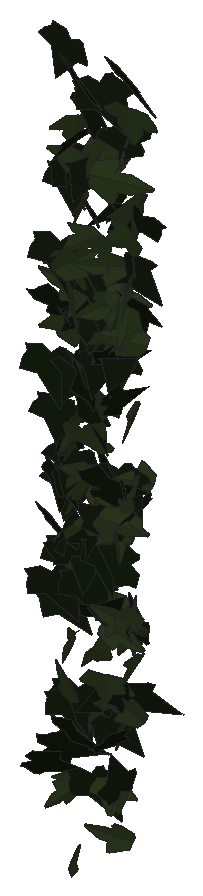
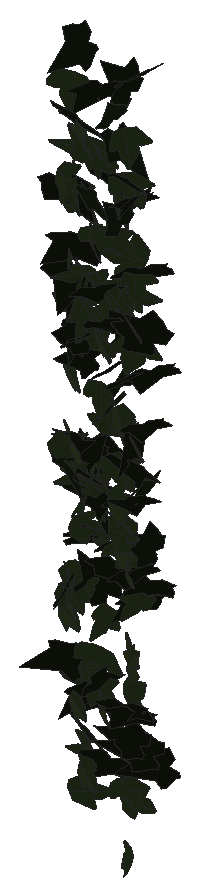
# SketchUp Ruby script. Lengths in inches.
U = 1.inch
M = Sketchup.active_model
def pt(a) = Geom::Point3d.new(a.map { |v| v * U })
def face(e, loops, mat)
  f = e.add_face(loops[0].map { |a| pt(a) })
  loops[1..].each { |l| e.add_face(l.map { |a| pt(a) }).erase! }
  f.material = f.back_material = mat if mat
  f
end
# faces: each face lists its corners as indices into pts; further lists are holes
def faces(e, pts, list, mat = nil) = list.each { |f| face(e, (f[0].is_a?(Array) ? f : [f]).map { |l| l.map { |i| pts[i] } }, mat) }
# xy, xz, yz: faces in a plane at the given z, y or x. An outline is a flat list of corners, or four numbers for a rectangle; further outlines are holes
def ring(l) = l.size == 4 ? [[l[0], l[1]], [l[2], l[1]], [l[2], l[3]], [l[0], l[3]]] : l.each_slice(2).to_a
def flat(e, list, mat, &to3) = list.each { |f| face(e, (f[0].is_a?(Array) ? f : [f]).map { |l| ring(l).map { |u, v| to3.(u, v) } }, mat) }
def xy(e, z, list, mat = nil) = flat(e, list, mat) { |x, y| [x, y, z] }
def xz(e, y, list, mat = nil) = flat(e, list, mat) { |x, z| [x, y, z] }
def yz(e, x, list, mat = nil) = flat(e, list, mat) { |y, z| [x, y, z] }
def lines(e, pts, list) = list.each { |a, b| e.add_line(pt(pts[a]), pt(pts[b])) }
# prism: a flat outline (further loops are holes) pulled along v
def prism(e, loops, v, mat = nil)
  f = face(e, loops, mat); d = Geom::Vector3d.new(v.map { |x| x * U })
  f.pushpull(f.normal.samedirection?(d) ? d.length : -d.length)
end
def box(e, o, s, mat = nil) = prism(e, [[o, [o[0] + s[0], o[1], o[2]], [o[0] + s[0], o[1] + s[1], o[2]], [o[0], o[1] + s[1], o[2]]]], [0, 0, s[2]], mat)
def at(x, y, z, deg = 0) = Geom::Transformation.translation(pt([x, y, z])) * Geom::Transformation.rotation(ORIGIN, Z_AXIS, deg.degrees)
def axes(o, x, y, z) = Geom::Transformation.new([*x, 0, *y, 0, *z, 0, *pt(o).to_a, 1])
def part(name) = M.definitions.add(name)
# library, detail: a bought-in or finely detailed component or shape, given as its bounding box
def library(name, o, s) = part(name).tap { |d| box(d.entities, o, s) }
def detail(e, o, s) = box(e.add_group.entities, o, s)
def put(e, d, t, mat = nil) = e.add_instance(d, t).tap { |i| i.material = mat if mat }
def group(e, t, mat = nil) = e.add_group.tap { |g| g.transformation = t; g.material = mat if mat }.entities
root = M.entities
M.materials.add("1026 AP 7946 SUNNY SIDE UP").color = [254, 231, 186]
M.materials.add("efeu1").color = [18, 25, 13]
M.materials.add("efeu2").color = [43, 57, 29]
c1 = part("ivyleaf_10")
p = [[0,0.5,-0.03],[-0.0625,2.02,-0.43],[-0.19,2.01,-0.46],[-0.54,1.05,-0.29],[-0.52,0.625,-0.18],[-0.83,0.76,-0.28],
  [-1.16,0.64,-0.33],[-1.15,0.33,-0.24],[-0.77,-0.39,0.02],[-0.3,-0.51,0.16],[0.04,-0.48,0.23],[-0.02,2.01,-0.4375],
  [-0.06,2.01,-0.43],[0.04,-0.49,0.23],[0.67,-0.49,0.14],[1.38,0.36,-0.2],[1.375,0.51,-0.24],[0.81,0.65,-0.19],
  [0.62,0.59,-0.15],[0.6,1.09,-0.28],[0.5,1.23,-0.31]]
faces(c1.entities,p,[[0,1,2,3,4,5,6,7,8,9,10],[11,12,0,13,14,15,16,17,18,19,20]],"efeu2")
c2 = part("ivyleaf_9")
p = [[1.54,2.16,1.25],[1.36,2.04,1.19],[-0.21,0.99,0.68],[-0.71,1.11,0.82],[-0.85,0.86,0.67],[-0.8,0.17,0.21],
  [-0.9,-0.01,0.1],[-0.67,-0.16,-0.02],[-0.08,-0.08,-0.05],[-0.03,-0.6,-0.4],[0.65,-0.88,-0.66],[0.83,-0.6,-0.49],
  [1.29,-0.42,-0.43],[1.8125,-0.07,-0.26],[1.21,0.44,0.15]]
faces(c2.entities,p,[[0,1,2,3,4,5,6,7,8,9,10,11,12,13,14]],"efeu1")
put(root,c1,axes([112.04,211.58,259.63],[-0.02218,-0.00666,0.26985],[0.14975,-0.24455,-0.00255],[0.38389,0.09501,0.01659]),"1026 AP 7946 SUNNY SIDE UP")
put(root,c2,axes([113.1,211.2,254.04],[0.15391,0.18308,0.14544],[0.11528,0.11962,-0.21306],[-0.34372,0.1221,-0.00633]),"1026 AP 7946 SUNNY SIDE UP")
put(root,c2,axes([113.43,211.23,253.19],[-0.30936,0.08367,-0.17603],[-0.22814,0.09407,0.2195],[0.19456,0.24335,-0.02252]),"1026 AP 7946 SUNNY SIDE UP")
put(root,c2,axes([112.72,211.41,259],[0.10094,0.00315,0.26449],[0.3707,-0.10549,-0.06002],[0.15983,0.24268,-0.02783]),"1026 AP 7946 SUNNY SIDE UP")
put(root,c2,axes([111.45,211.28,253.05],[0.27439,0.08812,0.17342],[0.25302,0.05173,-0.20003],[-0.15756,0.23652,-0.01922]),"1026 AP 7946 SUNNY SIDE UP")
put(root,c2,axes([111.625,211.52,261.22],[-0.10121,-0.2792,-0.08746],[0.02947,0.08118,-0.2947],[0.4572,-0.06704,-0.00036]),"1026 AP 7946 SUNNY SIDE UP")
put(root,c1,axes([113.27,211.5,252.01],[-0.09095,-0.01215,-0.2455],[-0.36534,-0.05265,0.06058],[-0.08495,0.23943,0.00233]),"1026 AP 7946 SUNNY SIDE UP")
put(root,c1,axes([113.06,211.34,258.47],[-0.13431,-0.07695,-0.25617],[0.36398,0.09625,-0.11223],[0.18576,-0.24423,0.03468]),"1026 AP 7946 SUNNY SIDE UP")
put(root,c1,axes([112.02,211.51,262.68],[-0.19608,0.22953,-0.16457],[0.09734,-0.14937,-0.26957],[-0.43001,-0.13848,0.01402]),"1026 AP 7946 SUNNY SIDE UP")
put(root,c2,axes([112.35,211.26,257.6],[-0.41504,0.13352,-0.08424],[-0.09726,0.05992,0.30403],[0.22684,0.26998,-0.02377]),"1026 AP 7946 SUNNY SIDE UP")
put(root,c2,axes([111.7,211.46,256.84],[-0.11315,-0.17882,-0.1991],[0.18009,0.15799,-0.19464],[0.3715,-0.13105,0.03372]),"1026 AP 7946 SUNNY SIDE UP")
put(root,c2,axes([111.68,211.64,258.74],[0.02999,-0.21354,0.17123],[0.00604,-0.16761,-0.22166],[0.42663,0.01739,-0.0089]),"1026 AP 7946 SUNNY SIDE UP")
put(root,c1,axes([113.03,211.4375,256.21],[0.11464,0.0422,0.24505],[0.36719,0.05035,-0.08273],[-0.09583,0.2434,-0.02384]),"1026 AP 7946 SUNNY SIDE UP")
put(root,c1,axes([113.3,211.4,253.03],[0.19212,-0.17785,-0.15897],[-0.15254,0.11914,-0.22135],[0.33622,0.15568,-0.00959]),"1026 AP 7946 SUNNY SIDE UP")
put(root,c2,axes([112.6875,211.5625,257.63],[0.04379,-0.2629,-0.01141],[-0.00693,0.00917,-0.27228],[0.4136,0.02799,-0.00336]),"1026 AP 7946 SUNNY SIDE UP")
put(root,c1,axes([113.31,211.55,262.59],[0.39846,-0.1214,0.07714],[0.08661,-0.05904,-0.28833],[0.20751,0.25776,-0.02779]),"1026 AP 7946 SUNNY SIDE UP")
put(root,c1,axes([113.01,211.58,263.48],[0.02748,0.00647,-0.26841],[-0.36284,-0.12107,-0.01975],[-0.19061,0.23141,-0.0011]),"1026 AP 7946 SUNNY SIDE UP")
put(root,c1,axes([113.32,211.51,258.93],[0.22626,-0.23331,-0.07497],[0.0778,-0.05332,0.28172],[-0.3757,-0.15155,0.01319]),"1026 AP 7946 SUNNY SIDE UP")
put(root,c2,axes([113.15,211.27,260.85],[0.06119,0.07554,0.25029],[0.27377,0.17072,-0.08257],[-0.29084,0.1766,-0.02506]),"1026 AP 7946 SUNNY SIDE UP")
put(root,c1,axes([113.34,211.5625,256.36],[-0.17491,-0.06534,-0.24772],[-0.35927,-0.07733,0.13028],[-0.15494,0.25306,-0.02244]),"1026 AP 7946 SUNNY SIDE UP")
put(root,c2,axes([112.3,211.62,257.53],[-0.10673,-0.26645,0.00292],[0.0045,-0.00521,-0.28327],[0.419,-0.06782,0.00378]),"1026 AP 7946 SUNNY SIDE UP")
put(root,c2,axes([112.42,211.51,256.98],[-0.164,-0.16956,-0.1863],[0.16946,0.14451,-0.20386],[0.34981,-0.1495,0.01142]),"1026 AP 7946 SUNNY SIDE UP")
put(root,c1,axes([113.48,211.6,262.07],[0.05756,0.07026,0.26662],[-0.25577,-0.20135,0.07896],[0.33449,-0.16605,0.01449]),"1026 AP 7946 SUNNY SIDE UP")
put(root,c2,axes([112.01,211.66,266.95],[0.14269,-0.16151,0.25112],[0.15557,-0.22424,-0.1916],[0.43395,0.1335,-0.01389]),"1026 AP 7946 SUNNY SIDE UP")
put(root,c1,axes([112.77,211.36,255.77],[-0.09376,-0.18861,-0.18934],[0.09541,0.17241,-0.20272],[0.40174,-0.08496,0.00396]),"1026 AP 7946 SUNNY SIDE UP")
put(root,c1,axes([113.45,211.6,260.7],[0.18456,-0.24275,0.09962],[0.05247,-0.09274,-0.27814],[0.40832,0.12164,-0.00929]),"1026 AP 7946 SUNNY SIDE UP")
put(root,c1,axes([112.11,211.31,263.27],[-0.0451,-0.13676,0.28314],[0.07044,0.272,0.14544],[-0.47864,0.05291,-0.00528]),"1026 AP 7946 SUNNY SIDE UP")
put(root,c1,axes([113.51,211.61,255.68],[0.04975,-0.21554,0.11849],[0.01456,-0.11607,-0.225],[0.38479,0.03226,-0.0068]),"1026 AP 7946 SUNNY SIDE UP")
put(root,c1,axes([112.85,211.45,265.29],[-0.00563,-0.0652,-0.31993],[0.49465,0.0372,-0.01158],[0.06094,-0.30796,0.06443]),"1026 AP 7946 SUNNY SIDE UP")
put(root,c1,axes([112.84,211.69,262.6],[0.08409,0.05383,-0.28802],[-0.25768,-0.22719,-0.0786],[-0.36668,0.172,-0.01082]),"1026 AP 7946 SUNNY SIDE UP")
put(root,c1,axes([112.4,211.61,259.1],[-0.22738,-0.19886,0.1324],[-0.08747,-0.1192,-0.25297],[0.36288,-0.15334,0.02199]),"1026 AP 7946 SUNNY SIDE UP")
put(root,c1,axes([112.5,211.53,259.78],[-0.38482,-0.04109,0.09426],[0.13978,0.0242,0.25564],[-0.07376,0.26024,-0.00732]),"1026 AP 7946 SUNNY SIDE UP")
put(root,c1,axes([111.93,211.62,259.73],[0.22835,-0.19183,0.08979],[0.06406,-0.07963,-0.24787],[0.32577,0.15012,-0.01419]),"1026 AP 7946 SUNNY SIDE UP")
put(root,c1,axes([113.4,211.5,264.22],[-0.24453,0.03139,0.20914],[-0.32189,-0.00541,-0.16087],[-0.02323,-0.25553,0.02758]),"1026 AP 7946 SUNNY SIDE UP")
put(root,c1,axes([112.97,211.57,252.9375],[0.3752,0.04405,0.02018],[0.03601,-0.01795,-0.24907],[-0.06653,0.23872,-0.021]),"1026 AP 7946 SUNNY SIDE UP")
put(root,c2,axes([112.64,211.53,256.32],[0.33869,0.12977,0.02203],[-0.04503,0.00767,0.25817],[0.20165,-0.21625,0.02066]),"1026 AP 7946 SUNNY SIDE UP")
put(root,c1,axes([113.1,211.6,258.12],[-0.02846,0.22322,-0.12106],[0.01378,-0.11846,-0.23141],[-0.39735,-0.0201,0.00065]),"1026 AP 7946 SUNNY SIDE UP")
put(root,c1,axes([113.22,211.59,258.7],[0.41399,-0.0452,-0.10964],[-0.17161,-0.01167,-0.27377],[0.05891,0.28364,-0.02703]),"1026 AP 7946 SUNNY SIDE UP")
put(root,c2,axes([111.79,211.52,256.48],[0.04527,-0.19567,-0.19128],[0.03036,0.18664,-0.19966],[0.42186,0.00757,0.03489]),"1026 AP 7946 SUNNY SIDE UP")
put(root,c2,axes([111.95,211.74,261.82],[-0.01217,-0.13586,0.2379],[0.13872,-0.22022,-0.13128],[0.39891,0.07244,0.05291]),"1026 AP 7946 SUNNY SIDE UP")
put(root,c2,axes([112.26,211.78,260.69],[-0.11172,-0.05878,0.27334],[-0.07183,-0.26809,-0.07526],[0.42175,-0.06123,0.05959]),"1026 AP 7946 SUNNY SIDE UP")
put(root,c2,axes([112.95,211.47,258.21],[-0.34215,0.02034,0.17623],[0.27063,0.01926,0.22344],[0.00633,0.27605,-0.02695]),"1026 AP 7946 SUNNY SIDE UP")
put(root,c1,axes([113.44,211.59,264.4],[-0.2305,0.2057,0.05092],[0.06399,-0.03016,0.25955],[0.326,0.15135,-0.01494]),"1026 AP 7946 SUNNY SIDE UP")
put(root,c2,axes([111.68,211.68,260.17],[-0.1405,-0.23919,-0.0491],[0.02635,0.04317,-0.2628],[0.38218,-0.09091,0.00007]),"1026 AP 7946 SUNNY SIDE UP")
put(root,c1,axes([113.1,211.62,262.25],[0.30775,-0.2433,-0.0362],[-0.05585,0.01468,-0.32103],[0.38217,0.19806,-0.01776]),"1026 AP 7946 SUNNY SIDE UP")
put(root,c2,axes([112.33,211.42,262.29],[-0.10707,0.2184,0.15919],[-0.08456,0.14372,-0.23472],[-0.41094,-0.08648,0.00682]),"1026 AP 7946 SUNNY SIDE UP")
put(root,c2,axes([113.08,211.62,259.32],[-0.15925,-0.1492,-0.20461],[0.23664,0.13265,-0.18172],[0.30941,-0.17824,0.03367]),"1026 AP 7946 SUNNY SIDE UP")
put(root,c2,axes([111.64,211.5,253.3],[0.18327,0.02019,0.24018],[0.36751,-0.00006,-0.12043],[-0.01412,0.26055,-0.01711]),"1026 AP 7946 SUNNY SIDE UP")
put(root,c1,axes([113.4,211.7,256.17],[-0.10942,-0.20613,0.11958],[-0.04406,-0.11418,-0.22461],[0.37027,-0.0745,0.00861]),"1026 AP 7946 SUNNY SIDE UP")
put(root,c1,axes([112.71,211.7,254.41],[-0.09429,-0.22143,0.11188],[-0.032,-0.10824,-0.23682],[0.38735,-0.06284,0.00767]),"1026 AP 7946 SUNNY SIDE UP")
put(root,c2,axes([113.07,211.57,267.5],[0.44822,-0.12414,-0.05396],[-0.08868,-0.00043,-0.31945],[0.19194,0.2897,-0.02159]),"1026 AP 7946 SUNNY SIDE UP")
put(root,c2,axes([112.08,211.78,260.98],[-0.16612,-0.20449,0.09169],[-0.04367,-0.08694,-0.23718],[0.34869,-0.10831,0.01398]),"1026 AP 7946 SUNNY SIDE UP")
put(root,c1,axes([112.25,211.65,264.52],[0.10419,-0.24391,0.01775],[-0.00015,-0.01931,-0.26044],[0.38464,0.06606,-0.00491]),"1026 AP 7946 SUNNY SIDE UP")
put(root,c1,axes([112.8,211.59,255.02],[-0.45319,-0.01634,-0.04731],[0.07441,-0.03017,-0.29569],[0.01777,-0.29027,0.03167]),"1026 AP 7946 SUNNY SIDE UP")
put(root,c2,axes([113.15,211.77,257.41],[-0.13407,-0.24512,-0.14438],[-0.08108,-0.12894,0.26655],[-0.43541,0.09949,-0.00518]),"1026 AP 7946 SUNNY SIDE UP")
put(root,c1,axes([111.98,211.56,257.32],[0.11102,-0.01553,-0.26424],[0.40225,0.0283,0.07097],[0.03653,-0.26444,0.02154]),"1026 AP 7946 SUNNY SIDE UP")
put(root,c2,axes([112.49,211.61,252.97],[-0.13245,-0.12284,-0.22839],[0.23434,0.16405,-0.1515],[0.32117,-0.17036,0.01635]),"1026 AP 7946 SUNNY SIDE UP")
put(root,c1,axes([111.86,211.76,252.4],[-0.05228,-0.11875,0.2008],[-0.05789,-0.19229,-0.12785],[0.35511,-0.04883,0.00872]),"1026 AP 7946 SUNNY SIDE UP")
put(root,c2,axes([112.36,211.73,260.3],[0.10743,-0.25465,0.03821],[0.00687,-0.03871,-0.27178],[0.40492,0.06822,-0.00553]),"1026 AP 7946 SUNNY SIDE UP")
put(root,c2,axes([111.82,211.625,258.79],[0.17564,-0.21305,-0.08843],[-0.0805,0.06858,-0.24707],[0.35136,0.12221,-0.0124]),"1026 AP 7946 SUNNY SIDE UP")
put(root,c1,axes([113.05,211.75,263.01],[0.32754,-0.14504,0.1643],[0.18119,-0.11386,-0.26105],[0.28762,0.23691,-0.02265]),"1026 AP 7946 SUNNY SIDE UP")
put(root,c1,axes([112.53,211.77,254.03],[0.14231,-0.07996,0.21829],[0.20913,-0.16653,-0.12397],[0.28906,0.15984,-0.01777]),"1026 AP 7946 SUNNY SIDE UP")
put(root,c1,axes([112.44,211.71,263.8125],[-0.22213,-0.08699,0.19607],[-0.22333,-0.12958,-0.16995],[0.24261,-0.19894,0.02308]),"1026 AP 7946 SUNNY SIDE UP")
put(root,c1,axes([113.34,211.62,266.66],[-0.46388,-0.00019,0.01272],[-0.01929,-0.0293,-0.30259],[0.00222,-0.29381,0.02843]),"1026 AP 7946 SUNNY SIDE UP")
put(root,c2,axes([112.04,211.73,259.29],[-0.36718,-0.09221,-0.12032],[0.18076,0.02469,-0.25787],[0.14757,-0.25969,0.01649]),"1026 AP 7946 SUNNY SIDE UP")
put(root,c1,axes([112.09,211.62,262.73],[-0.06583,-0.01384,-0.26069],[-0.39033,0.05347,0.03962],[0.0796,0.25077,-0.02129]),"1026 AP 7946 SUNNY SIDE UP")
put(root,c2,axes([112.69,211.84,254.58],[0.0069,-0.10624,-0.22872],[0.13024,-0.20783,0.10321],[-0.36353,-0.07648,0.03263]),"1026 AP 7946 SUNNY SIDE UP")
put(root,c2,axes([111.66,211.73,263.39],[-0.12418,-0.27694,-0.09736],[0.0577,0.0861,-0.29595],[0.45568,-0.08637,0.01094]),"1026 AP 7946 SUNNY SIDE UP")
put(root,c2,axes([112.24,211.83,266.34],[-0.00785,-0.21064,0.1636],[0.05608,-0.15911,-0.21557],[0.41214,0.01764,0.03245]),"1026 AP 7946 SUNNY SIDE UP")
put(root,c2,axes([112.24,211.65,265.9],[-0.15795,0.25238,-0.15154],[0.06135,-0.1441,-0.28026],[-0.45637,-0.10672,0.01477]),"1026 AP 7946 SUNNY SIDE UP")
put(root,c2,axes([113.5625,211.5,258.75],[-0.09048,0.25111,0.084],[-0.03984,0.07635,-0.26485],[-0.41254,-0.06245,0.00715]),"1026 AP 7946 SUNNY SIDE UP")
put(root,c1,axes([113.46,211.62,254.52],[-0.19768,0.01268,-0.22864],[-0.33636,0.06276,0.12885],[0.09551,0.24729,-0.01944]),"1026 AP 7946 SUNNY SIDE UP")
put(root,c1,axes([112.33,211.76,262.46],[-0.15523,-0.15216,0.15867],[-0.09617,-0.14376,-0.1865],[0.32758,-0.11431,0.02044]),"1026 AP 7946 SUNNY SIDE UP")
put(root,c2,axes([112.92,211.83,261.61],[-0.14352,-0.26704,0.04553],[-0.00759,-0.04662,-0.29081],[0.42594,-0.09081,0.01016]),"1026 AP 7946 SUNNY SIDE UP")
put(root,c2,axes([111.38,211.75,257.73],[0.23222,-0.15976,0.16517],[0.15513,-0.12806,-0.22456],[0.32143,0.17722,-0.01095]),"1026 AP 7946 SUNNY SIDE UP")
put(root,c2,axes([113.01,211.61,258.95],[0.13801,-0.14852,0.23433],[-0.11441,0.21837,0.17643],[-0.4127,-0.1102,0.02945]),"1026 AP 7946 SUNNY SIDE UP")
put(root,c1,axes([112.2,211.5625,257.93],[-0.16153,-0.12621,-0.18159],[0.20611,0.11821,-0.16588],[0.27036,-0.16552,0.01797]),"1026 AP 7946 SUNNY SIDE UP")
put(root,c1,axes([112.93,211.84,265.74],[-0.09131,0.01975,-0.27374],[0.11318,-0.26079,-0.03769],[-0.40357,-0.07761,0.05136]),"1026 AP 7946 SUNNY SIDE UP")
put(root,c2,axes([111.99,211.49,259.73],[0.0301,-0.04196,-0.29131],[-0.27789,0.22071,-0.04481],[0.35283,0.17741,-0.01044]),"1026 AP 7946 SUNNY SIDE UP")
put(root,c2,axes([112.9375,211.59,254.27],[0.022,-0.15416,-0.23039],[-0.02336,0.22228,-0.15814],[0.42533,0.02018,0.00323]),"1026 AP 7946 SUNNY SIDE UP")
put(root,c2,axes([111.74,211.73,253.57],[0.20267,-0.0685,0.20722],[0.24676,-0.12859,-0.14918],[0.22612,0.20172,-0.02293]),"1026 AP 7946 SUNNY SIDE UP")
put(root,c1,axes([113.49,211.84,259.16],[0.02272,0.09849,0.24176],[-0.06889,-0.23001,0.10113],[0.39338,-0.04597,0.00374]),"1026 AP 7946 SUNNY SIDE UP")
put(root,c1,axes([112,211.6,257.61],[0.20312,0.141,0.18435],[0.2213,0.11121,-0.19516],[-0.28044,0.18988,-0.02048]),"1026 AP 7946 SUNNY SIDE UP")
put(root,c1,axes([111.8,211.77,255.3],[0.06487,-0.20424,-0.10409],[0.0715,-0.09205,0.21272],[-0.35027,-0.05661,0.02414]),"1026 AP 7946 SUNNY SIDE UP")
put(root,c1,axes([112.02,211.6,254.48],[-0.23971,0.1351,-0.17683],[-0.18257,0.12829,0.21007],[0.29206,0.19108,-0.01383]),"1026 AP 7946 SUNNY SIDE UP")
put(root,c2,axes([112.88,211.7,261.5],[0.32634,0.20053,0.10751],[-0.14592,-0.05191,0.29584],[0.32322,-0.22591,0.02501]),"1026 AP 7946 SUNNY SIDE UP")
put(root,c1,axes([113.3,211.62,256.25],[0.23302,-0.18452,0.14097],[-0.11286,0.1188,0.24395],[-0.34417,-0.16389,0.01544]),"1026 AP 7946 SUNNY SIDE UP")
put(root,c1,axes([111.71,211.61,256.52],[0.11219,0.20213,0.14086],[0.09407,0.12239,-0.21969],[-0.37097,0.09216,-0.01311]),"1026 AP 7946 SUNNY SIDE UP")
put(root,c2,axes([112.8,211.66,258.41],[0.18371,-0.00878,-0.22961],[-0.34938,-0.02589,-0.11912],[-0.0297,0.25026,-0.01889]),"1026 AP 7946 SUNNY SIDE UP")
put(root,c1,axes([112.1,211.92,258.55],[0.07732,-0.15533,0.25408],[0.07427,-0.24347,-0.16849],[0.45344,0.06637,-0.01573]),"1026 AP 7946 SUNNY SIDE UP")
put(root,c1,axes([111.76,211.9,255.26],[0.0254,0.00619,0.27112],[0.20216,-0.23023,-0.00389],[0.36114,0.12844,-0.01689]),"1026 AP 7946 SUNNY SIDE UP")
put(root,c1,axes([112.08,211.56,251.05],[0.05657,-0.05491,0.23782],[-0.17548,0.20249,0.06863],[-0.32981,-0.11716,0.00428]),"1026 AP 7946 SUNNY SIDE UP")
put(root,c1,axes([112.01,211.74,266.02],[-0.18595,-0.2516,-0.00307],[0.01295,-0.00215,-0.28628],[0.39541,-0.11825,0.00793]),"1026 AP 7946 SUNNY SIDE UP")
put(root,c1,axes([112.17,211.73,260.23],[0.02099,-0.26389,-0.02971],[-0.0109,0.02702,-0.27199],[0.41702,0.01399,-0.00562]),"1026 AP 7946 SUNNY SIDE UP")
put(root,c2,axes([113.49,211.73,264.59],[0.11559,0.08063,-0.24591],[-0.28945,-0.15329,-0.11243],[-0.2715,0.19775,0.01516]),"1026 AP 7946 SUNNY SIDE UP")
put(root,c1,axes([113.2,211.88,256.06],[0.12437,-0.05986,0.2357],[0.24008,-0.17178,-0.10153],[0.28466,0.17103,-0.01735]),"1026 AP 7946 SUNNY SIDE UP")
put(root,c2,axes([111.6875,211.9375,267.43],[-0.13555,-0.23887,0.11899],[-0.01089,-0.12079,-0.26033],[0.418,-0.08061,0.03181]),"1026 AP 7946 SUNNY SIDE UP")
put(root,c2,axes([111.78,211.83,264.84],[-0.07589,-0.2476,-0.04357],[0.03533,0.03721,-0.25922],[0.39302,-0.05115,0.01489]),"1026 AP 7946 SUNNY SIDE UP")
put(root,c2,axes([113.4,211.54,261.47],[-0.11009,0.03489,-0.26612],[-0.3005,0.17533,0.07873],[0.27919,0.20247,-0.0202]),"1026 AP 7946 SUNNY SIDE UP")
put(root,c1,axes([111.78,211.74,263.25],[-0.16261,-0.22445,-0.03732],[0.04853,0.02416,-0.25379],[0.35386,-0.10645,0.01766]),"1026 AP 7946 SUNNY SIDE UP")
put(root,c1,axes([113.34,211.86,264.8],[0.01455,-0.24604,0.12115],[0.01216,-0.11878,-0.25433],[0.42958,0.0117,0.0031]),"1026 AP 7946 SUNNY SIDE UP")
put(root,c1,axes([112.875,211.7,262.03],[-0.24308,-0.19912,-0.09224],[0.11178,0.05637,-0.25852],[0.32382,-0.16893,0.02]),"1026 AP 7946 SUNNY SIDE UP")
put(root,c1,axes([112.54,211.81,261.73],[0.11753,-0.23624,0.04104],[0.0123,-0.04071,-0.25545],[0.37686,0.075,-0.00446]),"1026 AP 7946 SUNNY SIDE UP")
put(root,c1,axes([112.19,211.85,262.68],[-0.01921,-0.03916,0.24968],[0.35167,-0.10238,-0.00602],[0.16005,0.22026,0.0432]),"1026 AP 7946 SUNNY SIDE UP")
put(root,c1,axes([112.41,211.85,258.22],[-0.0396,0.18554,-0.1704],[0.03553,-0.16492,-0.19385],[-0.39033,-0.03384,-0.00035]),"1026 AP 7946 SUNNY SIDE UP")
put(root,c1,axes([113.21,211.8,264.58],[-0.11565,-0.23994,0.04599],[-0.01117,-0.04592,-0.25871],[0.38399,-0.0736,0.00632]),"1026 AP 7946 SUNNY SIDE UP")
put(root,c2,axes([112.41,211.9,262.13],[-0.25589,-0.1895,0.00976],[0.00982,-0.01924,-0.25683],[0.29827,-0.16194,0.01683]),"1026 AP 7946 SUNNY SIDE UP")
put(root,c2,axes([112.9375,211.77,264.61],[-0.26341,0.17583,-0.07053],[0.05509,-0.06232,-0.24995],[-0.29212,-0.1703,0.01646]),"1026 AP 7946 SUNNY SIDE UP")
put(root,c2,axes([111.83,211.79,254.25],[-0.10478,-0.17982,-0.16719],[0.16484,0.12918,-0.19226],[0.34216,-0.1173,0.04143]),"1026 AP 7946 SUNNY SIDE UP")
put(root,c1,axes([112,211.8,252.7],[-0.21874,-0.1761,0.05963],[-0.03999,-0.05481,-0.23109],[0.28921,-0.14076,0.01315]),"1026 AP 7946 SUNNY SIDE UP")
put(root,c2,axes([113.27,211.69,262.8],[0.40168,0.02162,-0.13922],[-0.20644,-0.04301,-0.26277],[-0.06145,0.28584,-0.02729]),"1026 AP 7946 SUNNY SIDE UP")
put(root,c1,axes([111.8,211.92,257.17],[0.06925,-0.047,0.24462],[0.2362,-0.18429,-0.06729],[0.29898,0.15648,-0.0035]),"1026 AP 7946 SUNNY SIDE UP")
put(root,c1,axes([113.01,211.7,265.42],[0.14496,-0.2764,0.11808],[-0.04328,0.11324,0.30068],[-0.46945,-0.09579,0.00874]),"1026 AP 7946 SUNNY SIDE UP")
put(root,c2,axes([112.33,211.95,261.17],[-0.07055,-0.23856,0.09168],[-0.01471,-0.09014,-0.2505],[0.40085,-0.04529,0.00695]),"1026 AP 7946 SUNNY SIDE UP")
put(root,c2,axes([112.54,211.78,266.89],[-0.0301,-0.24707,-0.1959],[0.05611,0.18612,-0.25361],[0.48567,-0.03682,0.01716]),"1026 AP 7946 SUNNY SIDE UP")
put(root,c1,axes([112.44,211.91,265.52],[-0.02276,-0.23375,0.145],[0.04719,-0.14278,-0.23967],[0.42752,0.00331,0.03418]),"1026 AP 7946 SUNNY SIDE UP")
put(root,c1,axes([112.64,211.92,263.71],[0.19431,-0.15268,0.18741],[0.18192,-0.14151,-0.20318],[0.32733,0.16928,0.00167]),"1026 AP 7946 SUNNY SIDE UP")
put(root,c1,axes([111.93,211.98,257.59],[0.08402,-0.11446,0.2545],[0.11734,-0.23665,-0.13062],[0.41269,0.09059,-0.01467]),"1026 AP 7946 SUNNY SIDE UP")
put(root,c1,axes([112.62,211.74,260.6],[-0.34636,0.10106,0.06081],[-0.09922,0.00197,-0.24845],[-0.15446,-0.22789,0.02323]),"1026 AP 7946 SUNNY SIDE UP")
put(root,c2,axes([111.4,211.79,262.05],[0.08458,-0.06025,0.28817],[0.41909,-0.09394,-0.07411],[0.16514,0.26927,0.04047]),"1026 AP 7946 SUNNY SIDE UP")
put(root,c2,axes([111.74,211.88,257.22],[-0.08268,-0.25668,-0.06401],[0.01606,0.05984,-0.26957],[0.41442,-0.05353,-0.00233]),"1026 AP 7946 SUNNY SIDE UP")
put(root,c1,axes([112.93,211.71,262.86],[-0.06167,-0.10043,-0.22275],[0.33413,0.08347,-0.07937],[0.16816,-0.20267,0.07602]),"1026 AP 7946 SUNNY SIDE UP")
put(root,c1,axes([113.05,211.9,254.09],[0.08972,-0.20515,0.10692],[0.04046,-0.10177,-0.21995],[0.36007,0.06255,-0.00192]),"1026 AP 7946 SUNNY SIDE UP")
put(root,c2,axes([111.86,211.94,258.67],[-0.23165,-0.22875,-0.01338],[0.02814,0.00236,-0.27993],[0.35905,-0.14777,0.0133]),"1026 AP 7946 SUNNY SIDE UP")
put(root,c1,axes([112.48,211.86,261.71],[0.30072,-0.01238,0.18885],[0.28322,-0.04006,-0.19654],[0.05754,0.26192,-0.01956]),"1026 AP 7946 SUNNY SIDE UP")
put(root,c1,axes([112.82,211.88,256.5],[0.09656,0.21733,-0.13799],[-0.04508,-0.1323,-0.23331],[-0.39991,0.06739,-0.00702]),"1026 AP 7946 SUNNY SIDE UP")
put(root,c1,axes([112.54,211.74,258.48],[0.28804,-0.03466,-0.14064],[0.22115,0.04877,0.1822],[0.00359,-0.22308,0.06029]),"1026 AP 7946 SUNNY SIDE UP")
put(root,c1,axes([113.06,211.62,262.49],[0.00267,-0.16899,-0.27388],[0.04893,0.26369,-0.17156],[0.49164,-0.02533,0.01856]),"1026 AP 7946 SUNNY SIDE UP")
put(root,c2,axes([113.47,211.76,256.02],[-0.08089,-0.18945,0.17418],[0.0972,0.1591,0.20268],[-0.38842,0.07927,0.01445]),"1026 AP 7946 SUNNY SIDE UP")
put(root,c2,axes([112.55,211.95,262.79],[-0.20623,-0.25856,-0.0231],[0.03348,0.01267,-0.29829],[0.40651,-0.13222,0.01285]),"1026 AP 7946 SUNNY SIDE UP")
put(root,c2,axes([112.22,211.92,265.22],[-0.37689,-0.09796,-0.09579],[0.15069,0.0085,-0.26528],[0.14879,-0.25675,0.02604]),"1026 AP 7946 SUNNY SIDE UP")
put(root,c2,axes([111.68,211.83,264.92],[0.09958,-0.22018,-0.10066],[-0.05634,0.08999,-0.23532],[0.37375,0.07223,-0.00866]),"1026 AP 7946 SUNNY SIDE UP")
put(root,c1,axes([112.9,211.97,257.79],[-0.04164,-0.06297,0.24287],[-0.12398,-0.22259,-0.07157],[0.36369,-0.08309,0.00341]),"1026 AP 7946 SUNNY SIDE UP")
put(root,c1,axes([111.74,211.79,261.84],[-0.33232,-0.15487,-0.05896],[0.08776,0.01897,-0.26923],[0.24382,-0.21791,0.01654]),"1026 AP 7946 SUNNY SIDE UP")
put(root,c1,axes([111.91,211.87,265.2],[-0.32606,-0.09916,0.11887],[-0.12211,-0.0998,-0.2316],[0.2065,-0.2156,0.05074]),"1026 AP 7946 SUNNY SIDE UP")
put(root,c2,axes([113.26,211.66,254.86],[0.0578,0.01936,-0.27639],[0.1193,0.25916,0.03147],[0.40597,-0.07891,0.0301]),"1026 AP 7946 SUNNY SIDE UP")
put(root,c2,axes([111.93,211.99,264.36],[0.08976,-0.1779,0.20594],[0.10196,-0.19018,-0.19357],[0.40947,0.08635,0.00305]),"1026 AP 7946 SUNNY SIDE UP")
put(root,c2,axes([113.37,211.78,266.04],[-0.28473,0.14249,0.15607],[-0.22695,0.05706,-0.23394],[-0.23417,-0.22856,0.03695]),"1026 AP 7946 SUNNY SIDE UP")
put(root,c1,axes([112.86,211.65,258.84],[-0.0223,0.10294,-0.23582],[-0.09132,0.2223,0.10773],[0.3848,0.05872,0.0119]),"1026 AP 7946 SUNNY SIDE UP")
put(root,c2,axes([111.94,211.89,254.4],[-0.22193,-0.16366,-0.15634],[0.17686,0.10167,-0.22147],[0.30198,-0.17982,0.01481]),"1026 AP 7946 SUNNY SIDE UP")
put(root,c1,axes([112.52,211.88,265.59],[0.37728,-0.04593,0.07138],[0.10042,-0.03486,-0.25091],[0.08421,0.24737,-0.02058]),"1026 AP 7946 SUNNY SIDE UP")
put(root,c2,axes([113.06,211.78,263.48],[-0.08203,-0.11095,-0.25528],[0.19636,0.21353,-0.12465],[0.37806,-0.13498,0.00935]),"1026 AP 7946 SUNNY SIDE UP")
put(root,c1,axes([112.83,211.91,252.79],[0.03744,-0.23425,0.06769],[0.00842,-0.06684,-0.24296],[0.38304,0.02437,-0.00128]),"1026 AP 7946 SUNNY SIDE UP")
put(root,c1,axes([113.3,211.72,263.41],[0.06091,-0.16624,-0.17911],[-0.02097,0.1734,-0.17379],[0.37658,0.03654,0.01929]),"1026 AP 7946 SUNNY SIDE UP")
